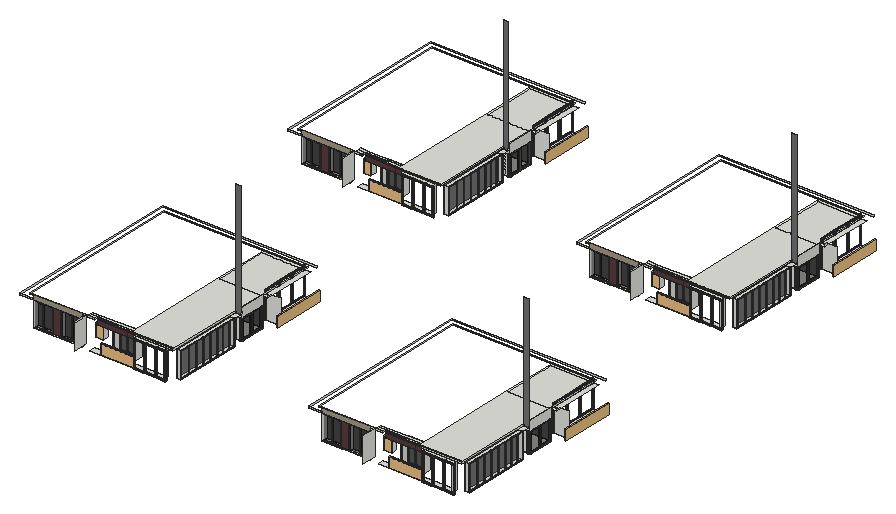
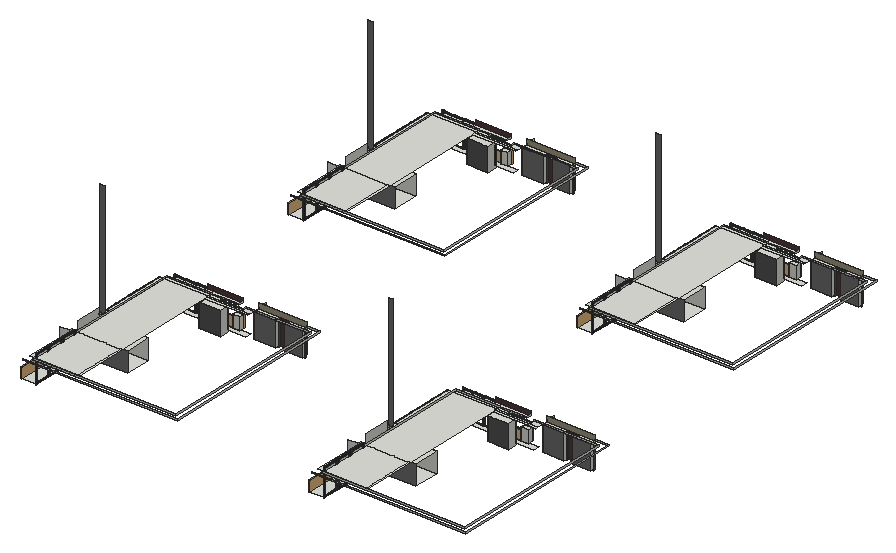
# SketchUp Ruby script. Lengths in inches.
U = 1.inch
M = Sketchup.active_model
def pt(a) = Geom::Point3d.new(a.map { |v| v * U })
def face(e, loops, mat)
  f = e.add_face(loops[0].map { |a| pt(a) })
  loops[1..].each { |l| e.add_face(l.map { |a| pt(a) }).erase! }
  f.material = f.back_material = mat if mat
  f
end
# faces: each face lists its corners as indices into pts; further lists are holes
def faces(e, pts, list, mat = nil) = list.each { |f| face(e, (f[0].is_a?(Array) ? f : [f]).map { |l| l.map { |i| pts[i] } }, mat) }
# xy, xz, yz: faces in a plane at the given z, y or x. An outline is a flat list of corners, or four numbers for a rectangle; further outlines are holes
def ring(l) = l.size == 4 ? [[l[0], l[1]], [l[2], l[1]], [l[2], l[3]], [l[0], l[3]]] : l.each_slice(2).to_a
def flat(e, list, mat, &to3) = list.each { |f| face(e, (f[0].is_a?(Array) ? f : [f]).map { |l| ring(l).map { |u, v| to3.(u, v) } }, mat) }
def xy(e, z, list, mat = nil) = flat(e, list, mat) { |x, y| [x, y, z] }
def xz(e, y, list, mat = nil) = flat(e, list, mat) { |x, z| [x, y, z] }
def yz(e, x, list, mat = nil) = flat(e, list, mat) { |y, z| [x, y, z] }
def lines(e, pts, list) = list.each { |a, b| e.add_line(pt(pts[a]), pt(pts[b])) }
# prism: a flat outline (further loops are holes) pulled along v
def prism(e, loops, v, mat = nil)
  f = face(e, loops, mat); d = Geom::Vector3d.new(v.map { |x| x * U })
  f.pushpull(f.normal.samedirection?(d) ? d.length : -d.length)
end
def box(e, o, s, mat = nil) = prism(e, [[o, [o[0] + s[0], o[1], o[2]], [o[0] + s[0], o[1] + s[1], o[2]], [o[0], o[1] + s[1], o[2]]]], [0, 0, s[2]], mat)
def at(x, y, z, deg = 0) = Geom::Transformation.translation(pt([x, y, z])) * Geom::Transformation.rotation(ORIGIN, Z_AXIS, deg.degrees)
def axes(o, x, y, z) = Geom::Transformation.new([*x, 0, *y, 0, *z, 0, *pt(o).to_a, 1])
def part(name) = M.definitions.add(name)
# library, detail: a bought-in or finely detailed component or shape, given as its bounding box
def library(name, o, s) = part(name).tap { |d| box(d.entities, o, s) }
def detail(e, o, s) = box(e.add_group.entities, o, s)
def put(e, d, t, mat = nil) = e.add_instance(d, t).tap { |i| i.material = mat if mat }
def group(e, t, mat = nil) = e.add_group.tap { |g| g.transformation = t; g.material = mat if mat }.entities
root = M.entities
M.materials.add("Glass_Tinted_Gray").color = [0, 0, 0]
M.materials["Glass_Tinted_Gray"].alpha = 0.125
M.materials.add("Glazing").color = [128, 128, 128]
M.materials["Glazing"].alpha = 0.05
M.materials.add("Powdercoating").color = [41, 44, 40]
M.materials.add("Wine2").color = [0, 0, 0]
M.materials["Wine2"].alpha = 0
M.materials.add("[0130_Gainsboro]").color = [39, 45, 50]
M.materials.add("[0135_DarkGray]").color = [81, 81, 81]
M.materials.add("[Color M05]").color = [114, 114, 114]
M.materials.add("[Color M06]").color = [86, 86, 86]
M.materials.add("[Concrete Tile]").color = [165, 155, 133]
M.materials.add("[Granite Brown]").color = [89, 59, 61]
M.materials.add("[Mirror 02]").color = [229, 229, 229]
M.materials.add("[Terrazzo Light Blue]").color = [196, 214, 227]
c1 = part("Framed glazing panel")
xy(c1.entities,0,[[0,-0.98,43.07,0],[0,0,43.07,1.4]],"[0130_Gainsboro]")
xy(c1.entities,0.3,[[0.3,-1.43,42.77,-0.98]],"[0130_Gainsboro]")
xy(c1.entities,2.95,[[2.95,-1.43,40.12,-0.63],[2.95,-0.63,40.12,0],[2.95,0,40.12,0.64],[2.95,0.64,40.12,1.4]],"[0130_Gainsboro]")
xy(c1.entities,3.54,[[3.54,-0.63,39.53,0],[3.54,0,39.53,0.64]],"[0130_Gainsboro]")
xy(c1.entities,111.8125,[[3.54,-0.63,39.53,0],[3.54,0,39.53,0.64]],"[0130_Gainsboro]")
xy(c1.entities,112.4,[[2.95,-1.43,40.12,-0.63],[2.95,-0.63,40.12,0],[2.95,0,40.12,0.64],[2.95,0.64,40.12,1.4]],"[0130_Gainsboro]")
xy(c1.entities,115.05,[[0.3,-1.43,42.77,-0.98]],"[0130_Gainsboro]")
xy(c1.entities,115.35,[[0,-0.98,43.07,0],[0,0,43.07,1.4]],"[0130_Gainsboro]")
xz(c1.entities,-1.43,[[[0.3,0.3,42.77,115.05],[2.95,2.95,40.12,112.4]]],"[0130_Gainsboro]")
xz(c1.entities,-0.98,[[[0,0,43.07,115.35],[0.3,0.3,42.77,115.05]]],"[0130_Gainsboro]")
xz(c1.entities,-0.63,[[[2.95,2.95,40.12,112.4],[3.54,3.54,39.53,111.8125]]],"[0130_Gainsboro]")
xz(c1.entities,0,[[3.54,3.54,39.53,111.8125]],"Wine2")
xz(c1.entities,0,[[[0,0,43.07,115.35],[2.95,2.95,40.12,112.4]],[[2.95,2.95,40.12,112.4],[3.54,3.54,39.53,111.8125]]],"[0130_Gainsboro]")
xz(c1.entities,0.64,[[[2.95,2.95,40.12,112.4],[3.54,3.54,39.53,111.8125]]],"[0130_Gainsboro]")
xz(c1.entities,1.4,[[[0,0,43.07,115.35],[2.95,2.95,40.12,112.4]]],"[0130_Gainsboro]")
yz(c1.entities,0,[[-0.98,0,0,115.35],[0,0,1.4,115.35]],"[0130_Gainsboro]")
yz(c1.entities,0.3,[[-1.43,0.3,-0.98,115.05]],"[0130_Gainsboro]")
yz(c1.entities,2.95,[[-1.43,2.95,-0.63,112.4],[-0.63,2.95,0,112.4],[0,2.95,0.64,112.4],[0.64,2.95,1.4,112.4]],"[0130_Gainsboro]")
yz(c1.entities,3.54,[[-0.63,3.54,0,111.8125],[0,3.54,0.64,111.8125]],"[0130_Gainsboro]")
yz(c1.entities,39.53,[[-0.63,3.54,0,111.8125],[0,3.54,0.64,111.8125]],"[0130_Gainsboro]")
yz(c1.entities,40.12,[[-1.43,2.95,-0.63,112.4],[-0.63,2.95,0,112.4],[0,2.95,0.64,112.4],[0.64,2.95,1.4,112.4]],"[0130_Gainsboro]")
yz(c1.entities,42.77,[[-1.43,0.3,-0.98,115.05]],"[0130_Gainsboro]")
yz(c1.entities,43.07,[[-0.98,0,0,115.35],[0,0,1.4,115.35]],"[0130_Gainsboro]")
c2 = part("Glazed panel assembly")
put(c2.entities,c1,axes([90.57,1.43,0],[1.05148,0,0],[0,1,0],[0,0,1]))
put(c2.entities,c1,axes([0,1.43,0],[1.05148,0,0],[0,1,0],[0,0,1]))
put(c2.entities,c1,axes([45.29,1.43,0],[1.05148,0,0],[0,1,0],[0,0,1]))
c3 = part("PENTEK_RP Fineline 50S_Sliding_DoorCase_E1")
box(c3.entities,[0,0,0],[1.51,3.66,99.27],"[0135_DarkGray]")
c4 = part("PENTEK_RP Fineline 50S_SlidingDooe_Case_E2")
box(c4.entities,[0,0,0],[96.25,3.66,1.51],"[0135_DarkGray]")
c5 = part("pentek_RP Fineline 50S_SlidingDoor_Case")
put(c5.entities,c3,at(97.76,0,0))
put(c5.entities,c4,at(1.51,0,0))
put(c5.entities,c3,at(0,0,0))
put(c5.entities,c4,at(1.51,0,97.76))
c6 = part("PENTEK_RP Fineline 50S_SlidingDoor_GlazingBead_2")
box(c6.entities,[0,0,0],[0.56,0.59,94.39],"[0135_DarkGray]")
c7 = part("PENTEK_RP Fineline 50S_SlidingDoor_Glass")
box(c7.entities,[0,0,0],[46.58,0.16,94.39],"Glass_Tinted_Gray")
c8 = part("PENTEK_RP Fineline 50S_SlidingDoor_GlazingBead")
box(c8.entities,[0,0,0],[45.47,0.59,0.56],"[0135_DarkGray]")
c9 = part("PENTEK_RP Fineline 50S_SlidingDoor_Leaf_E1")
xy(c9.entities,0,[[0,0,0.93,1.97],[0.93,1.57,1.49,1.97]],"[0135_DarkGray]")
xy(c9.entities,96.25,[[0,0,0.93,0,0.93,1.57,1.49,1.57,1.49,1.97,0,1.97]],"[0135_DarkGray]")
xz(c9.entities,0,[[0,0,0.93,96.25]],"[0135_DarkGray]")
xz(c9.entities,1.57,[[0.93,0,1.49,95.32],[0.93,95.32,1.49,96.25]],"[0135_DarkGray]")
xz(c9.entities,1.97,[[0,0,1.49,96.25]],"[0135_DarkGray]")
yz(c9.entities,0,[[0,0,1.97,96.25]],"[0135_DarkGray]")
yz(c9.entities,0.93,[[0,0,1.57,0.93],[0,0.93,1.57,95.32],[0,95.32,1.57,96.25]],"[0135_DarkGray]")
yz(c9.entities,1.49,[[1.57,0,1.97,95.32],[1.57,95.32,1.97,96.25]],"[0135_DarkGray]")
c10 = part("PENTEK_RP Fineline 50S_SlidingDoor_Leaf_E2")
xy(c10.entities,0,[[0,0,0,1.57,0.56,1.57,0.56,1.97,46.02,1.97,46.02,1.57,46.58,1.57,46.58,0]],"[0135_DarkGray]")
xy(c10.entities,0.93,[[0,0,46.58,1.57]],"[0135_DarkGray]")
xy(c10.entities,1.49,[[0.56,1.57,46.02,1.97]],"[0135_DarkGray]")
xz(c10.entities,0,[[0,0,46.58,0.93]],"[0135_DarkGray]")
xz(c10.entities,1.57,[[0,0,0.56,0.93],[46.02,0,46.58,0.93],[0.56,0.93,46.02,1.49]],"[0135_DarkGray]")
xz(c10.entities,1.97,[[0.56,0,46.02,1.49]],"[0135_DarkGray]")
yz(c10.entities,0,[[0,0,1.57,0.93]],"[0135_DarkGray]")
yz(c10.entities,0.56,[[1.57,0,1.97,0.93],[1.57,0.93,1.97,1.49]],"[0135_DarkGray]")
yz(c10.entities,46.02,[[1.57,0,1.97,0.93],[1.57,0.93,1.97,1.49]],"[0135_DarkGray]")
yz(c10.entities,46.58,[[0,0,1.57,0.93]],"[0135_DarkGray]")
c11 = part("PENTEK_RP Fineline S_SlidingDoor_Leaf1")
put(c11.entities,c6,at(0.93,0,0.93))
put(c11.entities,c6,at(46.96,0,0.93))
put(c11.entities,c7,at(1.49,1.42,0.93))
put(c11.entities,c8,at(1.49,0,0.93))
put(c11.entities,c7,at(1.49,0.59,0.93),"[Terrazzo Light Blue]")
put(c11.entities,c9,at(0,0,0))
put(c11.entities,c9,axes([48.44,0,0],[-1,0,0],[0,1,0],[0,0,1]))
put(c11.entities,c10,axes([0.93,0,96.25],[1,0,0],[0,1,0],[0,0,-1]))
put(c11.entities,c10,at(0.93,0,0))
put(c11.entities,c8,at(1.49,0,94.77))
c12 = part("PENTEK_RP Fineline 50S_SlidingDoor_Leaf2")
put(c12.entities,c7,at(1.49,1.42,0.93))
put(c12.entities,c8,at(1.49,0,94.77))
put(c12.entities,c6,at(46.96,0,0.93))
put(c12.entities,c7,at(1.49,0.59,0.93),"[Mirror 02]")
put(c12.entities,c6,at(0.93,0,0.93))
put(c12.entities,c9,at(0,0,0))
put(c12.entities,c9,axes([48.44,0,0],[-1,0,0],[0,1,0],[0,0,1]))
put(c12.entities,c8,at(1.49,0,0.93))
put(c12.entities,c10,axes([0.93,0,96.25],[1,0,0],[0,1,0],[0,0,-1]))
put(c12.entities,c10,at(0.93,0,0))
c13 = part("PENTEK - Slimmest Steel Sliding Door / Window\#1")
put(c13.entities,c5,at(0,-1.88,-0.09))
put(c13.entities,c11,at(1.51,-2.27,1.42))
put(c13.entities,c12,at(49.32,-0.3,1.42))
c14 = part("Group\#15")
xy(c14.entities,0,[[0,-55.94,0.71,45.94]])
xy(c14.entities,0.2,[[0,-55.94,0.47,45.94],[0.47,45.94,0.71,46.42]])
xy(c14.entities,2.36,[[0.47,-55.94,0.71,46.42]])
xz(c14.entities,-55.94,[[0,0,0.71,0,0.71,2.36,0.47,2.36,0.47,0.2,0,0.2]])
xz(c14.entities,45.94,[[0,0,0.71,0.2]])
xz(c14.entities,46.42,[[0.47,0.2,0.71,2.36]])
yz(c14.entities,0,[[-55.94,0,45.94,0.2]])
yz(c14.entities,0.47,[[-55.94,0.2,46.42,2.36]])
yz(c14.entities,0.71,[[-55.94,0,45.94,0,45.94,0.2,46.42,0.2,46.42,2.36,-55.94,2.36]])
c15 = part("Group\#7")
xy(c15.entities,0,[[0,-59.09,0.71,45.94]])
xy(c15.entities,0.2,[[0,-59.09,0.47,45.94],[0.47,45.94,0.71,46.42]])
xy(c15.entities,2.36,[[0.47,-59.09,0.71,46.42]])
xz(c15.entities,-59.09,[[0,0,0.71,0,0.71,2.36,0.47,2.36,0.47,0.2,0,0.2]])
xz(c15.entities,45.94,[[0,0,0.71,0.2]])
xz(c15.entities,46.42,[[0.47,0.2,0.71,2.36]])
yz(c15.entities,0,[[-59.09,0,45.94,0.2]])
yz(c15.entities,0.47,[[-59.09,0.2,46.42,2.36]])
yz(c15.entities,0.71,[[-59.09,0,45.94,0,45.94,0.2,46.42,0.2,46.42,2.36,-59.09,2.36]])
c16 = part("Group\#16")
prism(c16.entities,[[[0.47,-56.18,0.2],[0,-56.18,0.2],[0,-56.18,0],[0.71,-56.18,0],[0.71,-56.18,2.36],[0.47,-56.18,2.36]]],[0,28.68,0])
c17 = part("Group\#10")
box(c17.entities,[-0.73,0,0],[27.99,0.55,102.05])
c18 = part("Group\#18")
xy(c18.entities,0,[[0.47,-56.18,0.47,-55.47,0,-55.47,0,-28.21,1.18,-28.21,1.18,-56.18]])
xy(c18.entities,0.2,[[0.71,-56.18,1.18,-28.21],[0,-55.47,0.47,-28.21],[0.47,-28.21,0.71,-27.74]])
xy(c18.entities,2.36,[[0.47,-56.18,0.71,-27.74]])
xz(c18.entities,-56.18,[[0.47,0,1.18,0,1.18,0.2,0.71,0.2,0.71,2.36,0.47,2.36]])
xz(c18.entities,-55.47,[[0,0,0.47,0.2]])
xz(c18.entities,-28.21,[[0,0,1.18,0.2]])
xz(c18.entities,-27.74,[[0.47,0.2,0.71,2.36]])
yz(c18.entities,0,[[-55.47,0,-28.21,0.2]])
yz(c18.entities,0.47,[[-56.18,0,-55.47,0.2],[-56.18,0.2,-27.74,2.36]])
yz(c18.entities,0.71,[[-56.18,0.2,-27.74,2.36]])
yz(c18.entities,1.18,[[-56.18,0,-28.21,0.2]])
c19 = part("Group\#34")
xy(c19.entities,0,[[-20.45,0,7.76,1.22]])
xy(c19.entities,0.06,[[-20.39,0.06,7.7,1.22]])
xy(c19.entities,0.47,[[-19.98,0,7.28,0.06]])
xy(c19.entities,101.89,[[-19.98,0,7.28,0.06]])
xy(c19.entities,102.3,[[-20.39,0.06,7.7,1.22]])
xy(c19.entities,102.36,[[-20.45,0,7.76,1.22]])
xz(c19.entities,0,[[[-20.45,0,7.76,102.36],[-19.98,0.47,7.28,101.89]]])
xz(c19.entities,0.06,[[[-20.39,0.06,7.7,102.3],[-19.98,0.47,7.28,101.89]]])
xz(c19.entities,1.22,[[[-20.45,0,7.76,102.36],[-20.39,0.06,7.7,102.3]]])
yz(c19.entities,-20.45,[[0,0,1.22,102.36]])
yz(c19.entities,-20.39,[[0.06,0.06,1.22,102.3]])
yz(c19.entities,-19.98,[[0,0.47,0.06,101.89]])
yz(c19.entities,7.28,[[0,0.47,0.06,101.89]])
yz(c19.entities,7.7,[[0.06,0.06,1.22,102.3]])
yz(c19.entities,7.76,[[0,0,1.22,102.36]])
c20 = part("Group\#6")
put(c20.entities,c14,axes([27.97,0,7.875],[1,0,0],[0,0,-1],[0,1,0]),"Powdercoating")
put(c20.entities,c15,axes([0.71,0,6.8],[-1,0,0],[0,0,-0.97687],[0,1,0]),"Powdercoating")
put(c20.entities,c16,axes([-27.5,0,-38.07],[0,0,-1],[-1,0,0],[0,1,0]),"Powdercoating")
put(c20.entities,c17,at(1.12,0.35,-38.39),"Glazing")
put(c20.entities,c18,axes([-27.5,0,63.35],[0,0,1],[-1,0,0],[0,1,0]),"Powdercoating")
put(c20.entities,c19,at(20.6875,1.0625,-38.54),"Powdercoating")
c21 = part("Sliding door assembly")
put(c21.entities,c20,at(-1.18,4.5,38.86))
g1 = group(c21.entities,at(84.74,4.5,38.86))
put(g1,c14,axes([-27.97,0,7.875],[-1,0,0],[0,0,-1],[0,1,0]),"Powdercoating")
put(g1,c15,axes([-0.71,0,6.8],[1,0,0],[0,0,-0.97687],[0,1,0]),"Powdercoating")
put(g1,c16,axes([27.5,0,-38.07],[0,0,-1],[1,0,0],[0,1,0]),"Powdercoating")
put(g1,c17,axes([-1.12,0.35,-38.39],[-1,0,0],[0,1,0],[0,0,1]),"Glazing")
put(g1,c18,axes([27.5,0,63.35],[0,0,1],[1,0,0],[0,1,0]),"Powdercoating")
put(g1,c19,axes([-20.6875,1.0625,-38.54],[-1,0,0],[0,1,0],[0,0,1]),"Powdercoating")
g2 = group(c21.entities,at(56.0625,4.5,38.86))
put(g2,c14,axes([-27.97,0,7.875],[-1,0,0],[0,0,-1],[0,1,0]),"Powdercoating")
put(g2,c16,axes([27.5,0,-38.07],[0,0,-1],[1,0,0],[0,1,0]),"Powdercoating")
put(g2,c17,axes([-1.12,0.35,-38.39],[-1,0,0],[0,1,0],[0,0,1]),"Glazing")
put(g2,c18,axes([27.5,0,63.35],[0,0,1],[1,0,0],[0,1,0]),"Powdercoating")
put(g2,c19,axes([-20.6875,1.0625,-38.54],[-1,0,0],[0,1,0],[0,0,1]),"Powdercoating")
g3 = group(g2,at(-0.71,0,6.8),"Powdercoating")
xy(g3,-45.34,[[0.47,0.2,0.71,2.36]])
xy(g3,-44.88,[[0,0,0.71,0.2]])
xy(g3,57.73,[[0,0,0.71,0,0.71,2.36,0.47,2.36,0.47,0.2,0,0.2]])
xz(g3,0,[[0,-44.88,0.71,57.73]])
xz(g3,0.2,[[0.47,-45.34,0.71,-44.88],[0,-44.88,0.47,57.73]])
xz(g3,2.36,[[0.47,-45.34,0.71,57.73]])
yz(g3,0,[[0,-44.88,0.2,57.73]])
yz(g3,0.47,[[0.2,-45.34,2.36,57.73]])
yz(g3,0.71,[[0.2,-45.34,2.36,-45.34,2.36,57.73,0,57.73,0,-44.88,0.2,-44.88]])
put(c21.entities,c20,axes([-33.94,4.5,38.86],[1.14218,0,0],[0,1,0],[0,0,1]))
c22 = part("sliding door")
put(c22.entities,c21,at(0,-4.5,-0.08))
c23 = library("Glass Railing",[0,0,0],[139.5,4.76,42])
c24 = library("Klein+raam",[128.36,12.7,0],[19.68,5.51,55.12])
xy(root,1150.95,[[646.53,1835.1875,662.84,1873.375],[662.84,1835.1875,664.52,1873.375],[664.52,1835.1875,715.63,1873.375],[1864.72,1835.1875,1881.02,1873.375],[1881.02,1835.1875,1882.71,1873.375],
  [1882.71,1835.1875,1933.82,1873.375],[646.53,3249.875,662.84,3288.0625],[662.84,3249.875,664.52,3288.0625],[664.52,3249.875,715.63,3288.0625],[1864.72,3249.875,1881.02,3288.0625],
  [1881.02,3249.875,1882.71,3288.0625],[1882.71,3249.875,1933.82,3288.0625]])
xy(root,1151.26,[[625.7,1835.1875,646.53,1873.375],[1843.88,1835.1875,1864.72,1873.375],[625.7,3249.875,646.53,3288.0625],[1843.88,3249.875,1864.72,3288.0625]])
xy(root,1152.6875,[[557.88,1799.9375,869.48,1822.9375],[1776.07,1799.9375,2087.67,1822.9375],[894.3125,1835.1875,913.875,2117.96],[2112.5,1835.1875,2132.0625,2117.96],[557.88,3214.625,869.48,3237.625],
  [1776.07,3214.625,2087.67,3237.625],[894.3125,3249.875,913.875,3532.65],[2112.5,3249.875,2132.0625,3532.65]])
xy(root,1155.4375,[[319.53,1799.9375,404.32,1822.9375],[404.32,1799.9375,431.33,1806.5625],[431.33,1799.9375,523.04,1822.9375],[1537.72,1799.9375,1622.51,1822.9375],[1622.51,1799.9375,1649.52,1806.5625],
  [1649.52,1799.9375,1741.23,1822.9375],[319.53,3214.625,404.32,3237.625],[404.32,3214.625,431.33,3221.25],[431.33,3214.625,523.04,3237.625],[1537.72,3214.625,1622.51,3237.625],
  [1622.51,3214.625,1649.52,3221.25],[1649.52,3214.625,1741.23,3237.625]])
xy(root,1157.36,[[704.25,2156.01,913.875,2266.33],[1922.4375,2156.01,2132.0625,2266.33],[704.25,3570.7,913.875,3681.01],[1922.4375,3570.7,2132.0625,3681.01]])
xy(root,1160.8125,[[890.875,2310.68,954.6875,2518.89],[2109.0625,2310.68,2172.875,2518.89],[890.875,3725.37,954.6875,3933.57],[2109.0625,3725.37,2172.875,3933.57]])
xy(root,1189.98,[[557.4,1835.1875,588.66,1854.3125],[1775.59,1835.1875,1806.84,1854.3125],[557.4,3249.875,588.66,3269],[1775.59,3249.875,1806.84,3269]])
xy(root,1242.26,[[557.4,1835.1875,588.66,1854.3125],[1775.59,1835.1875,1806.84,1854.3125],[557.4,3249.875,588.66,3269],[1775.59,3249.875,1806.84,3269]])
xy(root,1243.04,[[704.25,2156.01,913.875,2266.33],[1922.4375,2156.01,2132.0625,2266.33],[704.25,3570.7,913.875,3681.01],[1922.4375,3570.7,2132.0625,3681.01]])
xy(root,1249.08,[[625.7,1835.1875,715.63,1873.375],[1843.88,1835.1875,1933.82,1873.375],[625.7,3249.875,715.63,3288.0625],[1843.88,3249.875,1933.82,3288.0625]])
xy(root,1260,[[319.53,1799.9375,319.53,1822.9375,404.92,1822.9375,404.92,1806.5625,431.33,1806.5625,431.33,1822.9375,523.04,1822.9375,523.04,1799.9375],[589.79,1799.9375,869.48,1822.9375],[1537.72,1799.9375,1537.72,1822.9375,1623.11,1822.9375,1623.11,1806.5625,1649.52,1806.5625,1649.52,1822.9375,1741.23,1822.9375,1741.23,1799.9375],[1807.98,1799.9375,2087.67,1822.9375],[523.04,1822.9375,557.4,1846],
  [653.67,1822.9375,704.25,1835.1875],[704.25,1822.9375,890.875,1835.1875],[1741.23,1822.9375,1775.59,1846],[1871.86,1822.9375,1922.4375,1835.1875],[1922.4375,1822.9375,2109.0625,1835.1875],
  [557.4,1835.1875,704.25,1846],[704.25,1835.1875,890.875,2295.875],[894.3125,1835.1875,913.875,2117.96],[1775.59,1835.1875,1922.4375,1846],[1922.4375,1835.1875,2109.0625,2295.875],
  [2112.5,1835.1875,2132.0625,2117.96],[523.04,1846,557.4,1856.375],[557.4,1846,704.25,1856.375],[1741.23,1846,1775.59,1856.375],[1775.59,1846,1922.4375,1856.375],
  [894.3125,2117.96,913.875,2148.83],[2112.5,2117.96,2132.0625,2148.83],[894.3125,2148.83,913.875,2156.01],[2112.5,2148.83,2132.0625,2156.01],[704.25,2295.875,710.125,2518.89],
  [710.125,2295.875,890.875,2518.89],[890.875,2295.875,913.875,2310.68],[1922.4375,2295.875,1928.3125,2518.89],[1928.3125,2295.875,2109.0625,2518.89],[2109.0625,2295.875,2132.0625,2310.68],
  [890.875,2310.68,913.875,2518.89],[2109.0625,2310.68,2132.0625,2518.89],[704.25,2518.89,890.875,2531.375],[1922.4375,2518.89,2109.0625,2531.375],[319.53,3214.625,319.53,3237.625,404.92,3237.625,404.92,3221.25,431.33,3221.25,431.33,3237.625,523.04,3237.625,523.04,3214.625],
  [589.79,3214.625,869.48,3237.625],[1537.72,3214.625,1537.72,3237.625,1623.11,3237.625,1623.11,3221.25,1649.52,3221.25,1649.52,3237.625,1741.23,3237.625,1741.23,3214.625],[1807.98,3214.625,2087.67,3237.625],[523.04,3237.625,557.4,3260.6875],[653.67,3237.625,704.25,3249.875],
  [704.25,3237.625,890.875,3249.875],[1741.23,3237.625,1775.59,3260.6875],[1871.86,3237.625,1922.4375,3249.875],[1922.4375,3237.625,2109.0625,3249.875],[557.4,3249.875,704.25,3260.6875],
  [704.25,3249.875,890.875,3710.5625],[894.3125,3249.875,913.875,3532.65],[1775.59,3249.875,1922.4375,3260.6875],[1922.4375,3249.875,2109.0625,3710.5625],[2112.5,3249.875,2132.0625,3532.65],
  [523.04,3260.6875,557.4,3271.0625],[557.4,3260.6875,704.25,3271.0625],[1741.23,3260.6875,1775.59,3271.0625],[1775.59,3260.6875,1922.4375,3271.0625],[894.3125,3532.65,913.875,3563.51],
  [2112.5,3532.65,2132.0625,3563.51],[894.3125,3563.51,913.875,3570.7],[2112.5,3563.51,2132.0625,3570.7],[704.25,3710.5625,710.125,3933.57],[710.125,3710.5625,890.875,3933.57],
  [890.875,3710.5625,913.875,3725.37],[1922.4375,3710.5625,1928.3125,3933.57],[1928.3125,3710.5625,2109.0625,3933.57],[2109.0625,3710.5625,2132.0625,3725.37],[890.875,3725.37,913.875,3933.57],
  [2109.0625,3725.37,2132.0625,3933.57],[704.25,3933.57,890.875,3946.0625],[1922.4375,3933.57,2109.0625,3946.0625]])
xy(root,1260,[[557.4,1822.9375,557.88,1835.1875],[1775.59,1822.9375,1776.07,1835.1875],[557.4,3237.625,557.88,3249.875],[1775.59,3237.625,1776.07,3249.875]],"[Granite Brown]")
xz(root,1799.9375,[[262.875,1260,319.53,1266],[1481.0625,1260,1537.72,1266]])
xz(root,1799.9375,[[319.53,1260,523.04,1281.4375],[1537.72,1260,1741.23,1281.4375]],"[Concrete Tile]")
xz(root,1799.9375,[[589.79,1260,736.96,1278.6875],[1807.98,1260,1955.15,1278.6875]],"[Granite Brown]")
xz(root,1806.5625,[[404.32,1155.4375,431.33,1155.4375,431.33,1260,404.92,1260,394.11,1260.05,393.59,1155.49],[1622.51,1155.4375,1649.52,1155.4375,1649.52,1260,1623.11,1260,1612.3,1260.05,1611.78,1155.49]],"[Granite Brown]")
xz(root,1822.9375,[[285.875,1260,285.875,1266,557.4,1266,557.4,1260,404.92,1260,394.11,1260.05,394.11,1260],[394.11,1260,394.11,1260.05,404.92,1260],[589.79,1260,653.67,1264.5625],[653.67,1260,653.67,1264.5625,704.25,1264.5625,704.25,1266,890.875,1266,890.875,1260],[1504.0625,1260,1504.0625,1266,1775.59,1266,1775.59,1260,1623.11,1260,1612.3,1260.05,1612.3,1260],
  [1612.3,1260,1612.3,1260.05,1623.11,1260],[1807.98,1260,1871.86,1264.5625],[1871.86,1260,1871.86,1264.5625,1922.4375,1264.5625,1922.4375,1266,2109.0625,1266,2109.0625,1260]])
xz(root,1822.9375,[[319.53,1155.4375,393.59,1155.4375,394.11,1260,319.53,1260],[431.33,1155.4375,523.04,1260],[1537.72,1155.4375,1611.78,1155.4375,1612.3,1260,1537.72,1260],[1649.52,1155.4375,1741.23,1260]],"[Color M05]")
xz(root,1822.9375,[[557.4,1260,557.88,1264.5625],[1775.59,1260,1776.07,1264.5625]],"[Granite Brown]")
xz(root,1835.1875,[[894.3125,1152.6875,913.875,1260],[2112.5,1152.6875,2132.0625,1260],[556.34,1189.98,557.4,1242.26],[1774.53,1189.98,1775.59,1242.26],[557.4,1260,653.67,1264.5625],
  [1775.59,1260,1871.86,1264.5625]])
xz(root,1835.1875,[[557.4,1189.98,557.88,1242.26],[1775.59,1189.98,1776.07,1242.26]],"[Granite Brown]")
xz(root,1854.3125,[[557.4,1189.98,588.66,1242.26],[1775.59,1189.98,1806.84,1242.26]])
xz(root,1873.375,[[646.53,1150.95,715.63,1150.95,715.63,1249.08,625.7,1249.08,625.7,1151.26,646.53,1151.26],[1864.72,1150.95,1933.82,1150.95,1933.82,1249.08,1843.88,1249.08,1843.88,1151.26,1864.72,1151.26]],"[Color M06]")
xz(root,2117.96,[[894.3125,1152.6875,913.875,1260],[2112.5,1152.6875,2132.0625,1260]])
xz(root,2148.83,[[894.3125,1260,913.875,1747.04],[2112.5,1260,2132.0625,1747.04]],"[Color M05]")
xz(root,2156.01,[[704.25,1157.36,894.3125,1243.04],[894.3125,1157.36,913.875,1243.04],[1922.4375,1157.36,2112.5,1243.04],[2112.5,1157.36,2132.0625,1243.04],[894.3125,1243.04,913.875,1260],
  [2112.5,1243.04,2132.0625,1260],[894.3125,1260,913.875,1266],[2112.5,1260,2132.0625,1266]])
xz(root,2266.33,[[704.25,1157.36,913.875,1243.04],[1922.4375,1157.36,2132.0625,1243.04]],"[Color M05]")
xz(root,2310.68,[[890.875,1160.8125,890.875,1260,913.875,1260,913.875,1266,954.6875,1266,954.6875,1160.8125],[2109.0625,1160.8125,2109.0625,1260,2132.0625,1260,2132.0625,1266,2172.875,1266,2172.875,1160.8125]])
xz(root,2531.375,[[285.875,1260,890.875,1266],[1504.0625,1260,2109.0625,1266]])
xz(root,2554.375,[[262.875,1260,913.875,1266],[1481.0625,1260,2132.0625,1266]])
xz(root,3214.625,[[262.875,1260,319.53,1266],[1481.0625,1260,1537.72,1266]])
xz(root,3214.625,[[319.53,1260,523.04,1281.4375],[1537.72,1260,1741.23,1281.4375]],"[Concrete Tile]")
xz(root,3214.625,[[589.79,1260,736.96,1278.6875],[1807.98,1260,1955.15,1278.6875]],"[Granite Brown]")
xz(root,3221.25,[[404.32,1155.4375,431.33,1155.4375,431.33,1260,404.92,1260,394.11,1260.05,393.59,1155.49],[1622.51,1155.4375,1649.52,1155.4375,1649.52,1260,1623.11,1260,1612.3,1260.05,1611.78,1155.49]],"[Granite Brown]")
xz(root,3237.625,[[285.875,1260,285.875,1266,557.4,1266,557.4,1260,404.92,1260,394.11,1260.05,394.11,1260],[394.11,1260,394.11,1260.05,404.92,1260],[589.79,1260,653.67,1264.5625],[653.67,1260,653.67,1264.5625,704.25,1264.5625,704.25,1266,890.875,1266,890.875,1260],[1504.0625,1260,1504.0625,1266,1775.59,1266,1775.59,1260,1623.11,1260,1612.3,1260.05,1612.3,1260],
  [1612.3,1260,1612.3,1260.05,1623.11,1260],[1807.98,1260,1871.86,1264.5625],[1871.86,1260,1871.86,1264.5625,1922.4375,1264.5625,1922.4375,1266,2109.0625,1266,2109.0625,1260]])
xz(root,3237.625,[[319.53,1155.4375,393.59,1155.4375,394.11,1260,319.53,1260],[431.33,1155.4375,523.04,1260],[1537.72,1155.4375,1611.78,1155.4375,1612.3,1260,1537.72,1260],[1649.52,1155.4375,1741.23,1260]],"[Color M05]")
xz(root,3237.625,[[557.4,1260,557.88,1264.5625],[1775.59,1260,1776.07,1264.5625]],"[Granite Brown]")
xz(root,3249.875,[[894.3125,1152.6875,913.875,1260],[2112.5,1152.6875,2132.0625,1260],[556.34,1189.98,557.4,1242.26],[1774.53,1189.98,1775.59,1242.26],[557.4,1260,653.67,1264.5625],
  [1775.59,1260,1871.86,1264.5625]])
xz(root,3249.875,[[557.4,1189.98,557.88,1242.26],[1775.59,1189.98,1776.07,1242.26]],"[Granite Brown]")
xz(root,3269,[[557.4,1189.98,588.66,1242.26],[1775.59,1189.98,1806.84,1242.26]])
xz(root,3288.0625,[[646.53,1150.95,715.63,1150.95,715.63,1249.08,625.7,1249.08,625.7,1151.26,646.53,1151.26],[1864.72,1150.95,1933.82,1150.95,1933.82,1249.08,1843.88,1249.08,1843.88,1151.26,1864.72,1151.26]],"[Color M06]")
xz(root,3532.65,[[894.3125,1152.6875,913.875,1260],[2112.5,1152.6875,2132.0625,1260]])
xz(root,3563.51,[[894.3125,1260,913.875,1747.04],[2112.5,1260,2132.0625,1747.04]],"[Color M05]")
xz(root,3570.7,[[704.25,1157.36,894.3125,1243.04],[894.3125,1157.36,913.875,1243.04],[1922.4375,1157.36,2112.5,1243.04],[2112.5,1157.36,2132.0625,1243.04],[894.3125,1243.04,913.875,1260],
  [2112.5,1243.04,2132.0625,1260],[894.3125,1260,913.875,1266],[2112.5,1260,2132.0625,1266]])
xz(root,3681.01,[[704.25,1157.36,913.875,1243.04],[1922.4375,1157.36,2132.0625,1243.04]],"[Color M05]")
xz(root,3725.37,[[890.875,1160.8125,890.875,1260,913.875,1260,913.875,1266,954.6875,1266,954.6875,1160.8125],[2109.0625,1160.8125,2109.0625,1260,2132.0625,1260,2132.0625,1266,2172.875,1266,2172.875,1160.8125]])
xz(root,3946.0625,[[285.875,1260,890.875,1266],[1504.0625,1260,2109.0625,1266]])
xz(root,3969.0625,[[262.875,1260,913.875,1266],[1481.0625,1260,2132.0625,1266]])
yz(root,262.875,[[1799.9375,1260,2554.375,1266],[3214.625,1260,3969.0625,1266]])
yz(root,285.875,[[1822.9375,1260,2531.375,1266],[3237.625,1260,3946.0625,1266]])
yz(root,319.53,[[1799.9375,1155.4375,1822.9375,1260],[3214.625,1155.4375,3237.625,1260]])
yz(root,431.33,[[1806.5625,1155.4375,1822.9375,1260],[3221.25,1155.4375,3237.625,1260]])
yz(root,523.04,[[1763.25,1155.4375,1822.9375,1260],[3177.9375,1155.4375,3237.625,1260],[1763.25,1260,1799.9375,1266],[3177.9375,1260,3214.625,1266]])
yz(root,557.4,[[1835.1875,1189.98,1854.3125,1242.26],[3249.875,1189.98,3269,1242.26],[1822.9375,1260,1835.1875,1264.5625],[3237.625,1260,3249.875,1264.5625]])
yz(root,588.66,[[1835.1875,1189.98,1854.3125,1242.26],[3249.875,1189.98,3269,1242.26]])
yz(root,589.79,[[1799.9375,1260,1822.9375,1266],[3214.625,1260,3237.625,1266]])
yz(root,625.7,[[1835.1875,1151.26,1873.375,1249.08],[3249.875,1151.26,3288.0625,1249.08]])
yz(root,646.53,[[1835.1875,1150.95,1873.375,1151.26],[3249.875,1150.95,3288.0625,1151.26]])
yz(root,653.67,[[1822.9375,1260,1835.1875,1264.5625],[3237.625,1260,3249.875,1264.5625]])
yz(root,715.63,[[1835.1875,1150.95,1873.375,1249.08],[3249.875,1150.95,3288.0625,1249.08]])
yz(root,869.48,[[1799.9375,1152.6875,1822.9375,1260],[3214.625,1152.6875,3237.625,1260]])
yz(root,890.875,[[1822.9375,1260,2531.375,1266],[3237.625,1260,3946.0625,1266]])
yz(root,894.3125,[[2148.83,1260,2156.01,1266],[3563.51,1260,3570.7,1266]])
yz(root,894.3125,[[1835.1875,1152.6875,2117.96,1260],[3249.875,1152.6875,3532.65,1260]],"[Color M05]")
yz(root,913.875,[[2156.01,1243.04,2266.33,1283.36],[3570.7,1243.04,3681.01,1283.36],[2148.83,1260,2156.01,1266],[2295.875,1260,2310.68,1266],[3563.51,1260,3570.7,1266],
  [3710.5625,1260,3725.37,1266]])
yz(root,1481.0625,[[1799.9375,1260,2554.375,1266],[3214.625,1260,3969.0625,1266]])
yz(root,1504.0625,[[1822.9375,1260,2531.375,1266],[3237.625,1260,3946.0625,1266]])
yz(root,1537.72,[[1799.9375,1155.4375,1822.9375,1260],[3214.625,1155.4375,3237.625,1260]])
yz(root,1649.52,[[1806.5625,1155.4375,1822.9375,1260],[3221.25,1155.4375,3237.625,1260]])
yz(root,1741.23,[[1763.25,1155.4375,1822.9375,1260],[3177.9375,1155.4375,3237.625,1260],[1763.25,1260,1799.9375,1266],[3177.9375,1260,3214.625,1266]])
yz(root,1775.59,[[1835.1875,1189.98,1854.3125,1242.26],[3249.875,1189.98,3269,1242.26],[1822.9375,1260,1835.1875,1264.5625],[3237.625,1260,3249.875,1264.5625]])
yz(root,1806.84,[[1835.1875,1189.98,1854.3125,1242.26],[3249.875,1189.98,3269,1242.26]])
yz(root,1807.98,[[1799.9375,1260,1822.9375,1266],[3214.625,1260,3237.625,1266]])
yz(root,1843.88,[[1835.1875,1151.26,1873.375,1249.08],[3249.875,1151.26,3288.0625,1249.08]])
yz(root,1864.72,[[1835.1875,1150.95,1873.375,1151.26],[3249.875,1150.95,3288.0625,1151.26]])
yz(root,1871.86,[[1822.9375,1260,1835.1875,1264.5625],[3237.625,1260,3249.875,1264.5625]])
yz(root,1933.82,[[1835.1875,1150.95,1873.375,1249.08],[3249.875,1150.95,3288.0625,1249.08]])
yz(root,2087.67,[[1799.9375,1152.6875,1822.9375,1260],[3214.625,1152.6875,3237.625,1260]])
yz(root,2109.0625,[[1822.9375,1260,2531.375,1266],[3237.625,1260,3946.0625,1266]])
yz(root,2112.5,[[2148.83,1260,2156.01,1266],[3563.51,1260,3570.7,1266]])
yz(root,2112.5,[[1835.1875,1152.6875,2117.96,1260],[3249.875,1152.6875,3532.65,1260]],"[Color M05]")
yz(root,2132.0625,[[2156.01,1243.04,2266.33,1283.36],[3570.7,1243.04,3681.01,1283.36],[2148.83,1260,2156.01,1266],[2295.875,1260,2310.68,1266],[3563.51,1260,3570.7,1266],
  [3710.5625,1260,3725.37,1266]])
p = [[404.92,1806.5625,1260],[404.92,1822.9375,1260],[394.11,1822.9375,1260.05],[394.11,1806.5625,1260.05],[1623.11,1806.5625,1260],[1623.11,1822.9375,1260],
  [1612.3,1822.9375,1260.05],[1612.3,1806.5625,1260.05],[404.92,3221.25,1260],[404.92,3237.625,1260],[394.11,3237.625,1260.05],[394.11,3221.25,1260.05],
  [1623.11,3221.25,1260],[1623.11,3237.625,1260],[1612.3,3237.625,1260.05],[1612.3,3221.25,1260.05],[1933.82,1799.9375,1260],[1933.82,1799.9375,1278.625],
  [715.63,1799.9375,1260],[715.63,1799.9375,1278.625],[1933.82,3214.625,1260],[1933.82,3214.625,1278.625],[715.63,3214.625,1260],[715.63,3214.625,1278.625]]
faces(root,p,[[0,1,2,3],[4,5,6,7],[8,9,10,11],[12,13,14,15]])
lines(root,p,[[16,17],[18,19],[20,21],[22,23]])
put(root,c2,at(1962.125,1797.87,1149.15))
put(root,c2,at(743.9375,1797.87,1149.15))
put(root,c2,at(1962.125,3212.55,1149.15))
put(root,c2,at(743.9375,3212.55,1149.15))
put(root,c13,axes([1646.7,1808.5625,1152.375],[0.94111,0,0],[0,0.88,0],[0,0,1.054]))
put(root,c13,axes([428.51,1808.5625,1152.375],[0.94111,0,0],[0,0.88,0],[0,0,1.054]))
put(root,c13,axes([1646.7,3223.25,1152.375],[0.94111,0,0],[0,0.88,0],[0,0,1.054]))
put(root,c13,axes([428.51,3223.25,1152.375],[0.94111,0,0],[0,0.88,0],[0,0,1.054]))
put(root,c13,axes([1534.89,1808.5625,1152.375],[0.77709,0,0],[0,0.88,0],[0,0,1.054]))
put(root,c13,axes([316.71,1808.5625,1152.375],[0.77709,0,0],[0,0.88,0],[0,0,1.054]))
put(root,c13,axes([1534.89,3223.25,1152.375],[0.77709,0,0],[0,0.88,0],[0,0,1.054]))
put(root,c13,axes([316.71,3223.25,1152.375],[0.77709,0,0],[0,0.88,0],[0,0,1.054]))
put(root,c22,axes([2132.0625,1879.38,1152.6875],[0,1.302,0],[-1,0,0],[0,0,1.03877]))
put(root,c22,axes([2132.0625,2028.24,1152.6875],[0,1.06764,0],[-1,0,0],[0,0,1.03877]))
put(root,c22,axes([913.875,2028.24,1152.6875],[0,1.06764,0],[-1,0,0],[0,0,1.03877]))
put(root,c22,axes([913.875,1879.38,1152.6875],[0,1.302,0],[-1,0,0],[0,0,1.03877]))
put(root,c22,axes([2132.0625,3442.93,1152.6875],[0,1.06764,0],[-1,0,0],[0,0,1.03877]))
put(root,c22,axes([2132.0625,3294.06,1152.6875],[0,1.302,0],[-1,0,0],[0,0,1.03877]))
put(root,c22,axes([913.875,3442.93,1152.6875],[0,1.06764,0],[-1,0,0],[0,0,1.03877]))
put(root,c22,axes([913.875,3294.06,1152.6875],[0,1.302,0],[-1,0,0],[0,0,1.03877]))
put(root,c23,at(1822.95,1797.87,1154.37))
put(root,c23,at(604.76,1797.87,1154.37))
put(root,c23,at(1822.95,3212.55,1154.37))
put(root,c23,at(604.76,3212.55,1154.37))
put(root,c13,axes([2127.34,2156.65,1156.11],[0,1.12181,0],[-2.51374,0,0],[0,0,0.87918]))
put(root,c13,axes([909.16,2156.65,1156.11],[0,1.12181,0],[-2.51374,0,0],[0,0,0.87918]))
put(root,c13,axes([2127.34,3571.34,1156.11],[0,1.12181,0],[-2.51374,0,0],[0,0,0.87918]))
put(root,c13,axes([909.16,3571.34,1156.11],[0,1.12181,0],[-2.51374,0,0],[0,0,0.87918]))
put(root,c2,axes([2109.0625,2310.05,1160.51],[0,1.54079,0],[-1,0,0],[0,0,1]))
put(root,c2,axes([890.875,2310.05,1160.51],[0,1.54079,0],[-1,0,0],[0,0,1]))
put(root,c2,axes([2109.0625,3724.73,1160.51],[0,1.54079,0],[-1,0,0],[0,0,1]))
put(root,c2,axes([890.875,3724.73,1160.51],[0,1.54079,0],[-1,0,0],[0,0,1]))
put(root,c23,axes([2172.875,2295.6875,1160.8125],[0,1.6,0],[-1,0,0],[0,0,1]))
put(root,c23,axes([954.6875,2295.6875,1160.8125],[0,1.6,0],[-1,0,0],[0,0,1]))
put(root,c23,axes([2172.875,3710.375,1160.8125],[0,1.6,0],[-1,0,0],[0,0,1]))
put(root,c23,axes([954.6875,3710.375,1160.8125],[0,1.6,0],[-1,0,0],[0,0,1]))
put(root,c2,axes([1843.49,1835.1875,1162.58],[0.6649,0,0],[0,0.61,0],[0,0,0.74986]),"[Color M06]")
put(root,c2,axes([625.3,1835.1875,1162.58],[0.6649,0,0],[0,0.61,0],[0,0,0.74986]),"[Color M06]")
put(root,c2,axes([1843.49,3249.875,1162.58],[0.6649,0,0],[0,0.61,0],[0,0,0.74986]),"[Color M06]")
put(root,c2,axes([625.3,3249.875,1162.58],[0.6649,0,0],[0,0.61,0],[0,0,0.74986]),"[Color M06]")
put(root,c24,axes([1571.78,1822.81,1189.98],[1.58777,0,0],[0,0.68,0],[0,0,0.99202]))
put(root,c24,axes([353.6,1822.81,1189.98],[1.58777,0,0],[0,0.68,0],[0,0,0.99202]))
put(root,c24,axes([1571.78,3237.49,1189.98],[1.58777,0,0],[0,0.68,0],[0,0,0.99202]))
put(root,c24,axes([353.6,3237.49,1189.98],[1.58777,0,0],[0,0.68,0],[0,0,0.99202]))
